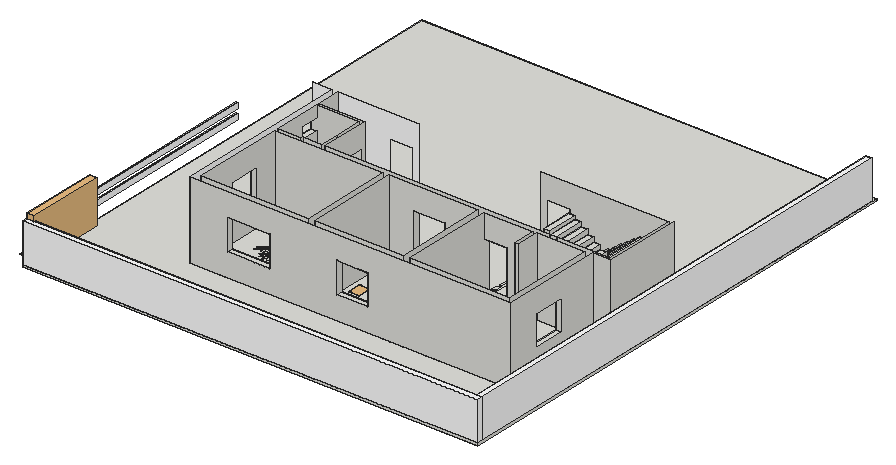
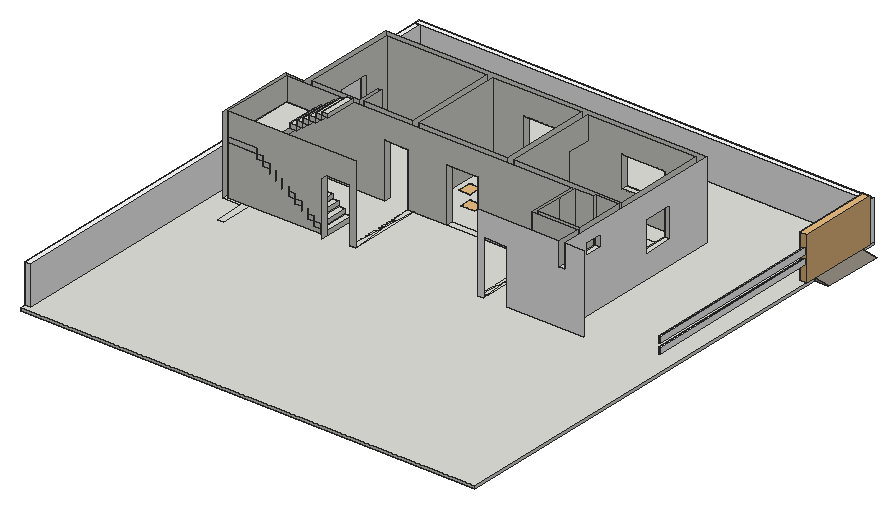
# SketchUp Ruby script. Lengths in inches.
U = 1.inch
M = Sketchup.active_model
def pt(a) = Geom::Point3d.new(a.map { |v| v * U })
def face(e, loops, mat)
  f = e.add_face(loops[0].map { |a| pt(a) })
  loops[1..].each { |l| e.add_face(l.map { |a| pt(a) }).erase! }
  f.material = f.back_material = mat if mat
  f
end
# faces: each face lists its corners as indices into pts; further lists are holes
def faces(e, pts, list, mat = nil) = list.each { |f| face(e, (f[0].is_a?(Array) ? f : [f]).map { |l| l.map { |i| pts[i] } }, mat) }
# xy, xz, yz: faces in a plane at the given z, y or x. An outline is a flat list of corners, or four numbers for a rectangle; further outlines are holes
def ring(l) = l.size == 4 ? [[l[0], l[1]], [l[2], l[1]], [l[2], l[3]], [l[0], l[3]]] : l.each_slice(2).to_a
def flat(e, list, mat, &to3) = list.each { |f| face(e, (f[0].is_a?(Array) ? f : [f]).map { |l| ring(l).map { |u, v| to3.(u, v) } }, mat) }
def xy(e, z, list, mat = nil) = flat(e, list, mat) { |x, y| [x, y, z] }
def xz(e, y, list, mat = nil) = flat(e, list, mat) { |x, z| [x, y, z] }
def yz(e, x, list, mat = nil) = flat(e, list, mat) { |y, z| [x, y, z] }
def lines(e, pts, list) = list.each { |a, b| e.add_line(pt(pts[a]), pt(pts[b])) }
# prism: a flat outline (further loops are holes) pulled along v
def prism(e, loops, v, mat = nil)
  f = face(e, loops, mat); d = Geom::Vector3d.new(v.map { |x| x * U })
  f.pushpull(f.normal.samedirection?(d) ? d.length : -d.length)
end
def box(e, o, s, mat = nil) = prism(e, [[o, [o[0] + s[0], o[1], o[2]], [o[0] + s[0], o[1] + s[1], o[2]], [o[0], o[1] + s[1], o[2]]]], [0, 0, s[2]], mat)
def at(x, y, z, deg = 0) = Geom::Transformation.translation(pt([x, y, z])) * Geom::Transformation.rotation(ORIGIN, Z_AXIS, deg.degrees)
def axes(o, x, y, z) = Geom::Transformation.new([*x, 0, *y, 0, *z, 0, *pt(o).to_a, 1])
def part(name) = M.definitions.add(name)
# library, detail: a bought-in or finely detailed component or shape, given as its bounding box
def library(name, o, s) = part(name).tap { |d| box(d.entities, o, s) }
def detail(e, o, s) = box(e.add_group.entities, o, s)
def put(e, d, t, mat = nil) = e.add_instance(d, t).tap { |i| i.material = mat if mat }
def group(e, t, mat = nil) = e.add_group.tap { |g| g.transformation = t; g.material = mat if mat }.entities
root = M.entities
M.materials.add("Manhattan Creative Coating MD 1125B 26.44cm").color = [255, 255, 255]
M.materials.add("Pp-1846-msg 17.72cm").color = [255, 255, 255]
M.materials.add("Tiles L02 200cm").color = [152, 144, 134]
c1 = library("Group\#36",[0,0,0],[178.08,17.07,78.35])
c2 = library("Chair - Desk\#3",[-10.5,-17,0],[21,17,0.01])
c3 = part("*U14\#2")
p = [[0,9.17,0],[-0.57,7.9375,0],[-1.06,6.67,0],[-1.46,5.37,0],[-1.77,4.05,0],[-1.99,2.71,0],
  [-2.13,1.36,0],[-2.17,0,0],[-2.13,-1.36,0],[-1.99,-2.71,0],[-1.77,-4.05,0],[-1.46,-5.37,0],
  [-1.06,-6.67,0],[-0.57,-7.9375,0],[0,-9.17,0],[0.57,-7.9375,0],[1.06,-6.67,0],[1.46,-5.37,0],
  [1.77,-4.05,0],[1.99,-2.71,0],[2.13,-1.36,0],[2.17,0,0],[2.13,1.36,0],[1.99,2.71,0],
  [1.77,4.05,0],[1.46,5.37,0],[1.06,6.67,0],[0.57,7.9375,0]]
lines(c3.entities,p,[[0,1],[1,2],[2,3],[3,4],[4,5],[5,6],[6,7],[7,8],[8,9],[9,10],[10,11],[11,12],
  [12,13],[13,14],[14,15],[15,16],[16,17],[17,18],[18,19],[19,20],[20,21],[21,22],[22,23],[23,24],
  [24,25],[25,26],[26,27],[27,0]])
c4 = part("*U15\#1")
put(c4.entities,c3,at(3814.69,2754.15,0))
put(c4.entities,c3,at(3810.96,2753.36,0,24))
put(c4.entities,c3,at(3807.875,2751.12,0,48))
put(c4.entities,c3,at(3805.97,2747.8125,0,72))
put(c4.entities,c3,at(3805.57,2744.02,0,96))
put(c4.entities,c3,at(3806.75,2740.39,0,120))
put(c4.entities,c3,at(3809.3,2737.56,0,144))
put(c4.entities,c3,at(3812.79,2736.01,0,168))
put(c4.entities,c3,at(3816.6,2736.01,0,-168))
put(c4.entities,c3,at(3820.09,2737.56,0,-144))
put(c4.entities,c3,at(3822.64,2740.39,0,-120))
put(c4.entities,c3,at(3823.82,2744.02,0,-96))
put(c4.entities,c3,at(3823.42,2747.8125,0,-72))
put(c4.entities,c3,at(3821.51,2751.12,0,-48))
put(c4.entities,c3,at(3818.42,2753.36,0,-24))
c5 = part("Group\#35")
box(c5.entities,[-3,0,0],[3,280.875,9])
c6 = library("*U30\#2",[-10.5,-33,0],[21,33,0.01])
c7 = part("Stair tread")
box(c7.entities,[0,0,0],[9.89,48,7])
c8 = part("Group\#5")
box(c8.entities,[108.84,0,77],[43.96,112.5,7])
xy(c8.entities,124,[[49.47,0,59.37,48]])
xz(c8.entities,48,[[49.47,119,59.37,124]])
yz(c8.entities,49.47,[[0,119,48,124]])
put(c8.entities,c7,at(9.89,64.5,7))
put(c8.entities,c7,at(19.79,64.5,14))
put(c8.entities,c7,at(0,64.5,0))
put(c8.entities,c7,at(29.68,64.5,21))
put(c8.entities,c7,at(39.58,64.5,28))
put(c8.entities,c7,at(49.47,64.5,35))
put(c8.entities,c7,at(89.05,64.5,63))
put(c8.entities,c7,at(89.05,0,91))
put(c8.entities,c7,at(79.16,0,98))
put(c8.entities,c7,at(98.95,64.5,70))
put(c8.entities,c7,at(69.26,0,105))
put(c8.entities,c7,at(79.16,64.5,56))
put(c8.entities,c7,at(59.37,64.5,42))
put(c8.entities,c7,at(69.26,64.5,49))
put(c8.entities,c7,at(98.95,0,84))
put(c8.entities,c7,at(59.37,0,112))
xy(root,0,[[178.31,129,178.31,199.58,187.31,199.58,187.31,138,236.56,138,236.56,129],[236.56,129,302.56,138],[302.56,129,302.56,138,502.31,138,502.31,282,481.31,282,481.31,291,511.31,291,511.31,138,667.31,138,667.31,175.67,676.31,175.67,676.31,129],[273.14,138,273.21,138,273.27,138.01,273.34,138.02,273.4,138.03,273.46,138.05,273.52,138.08,273.58,138.1,273.64,138.13,273.7,138.17,273.85,138.29,273.97,138.44,274.01,138.5,274.04,138.56,274.0625,138.62,274.09,138.68,274.11,138.74,274.12,138.8,274.13,138.87,274.14,138.93,274.14,167.08,274.13,167.17,274.09,167.35,274.07,167.4375,274.04,167.52,273.96,167.68,273.86,167.84,273.8,167.91,273.74,167.97,273.68,168.04,273.61,168.1,273.53,168.15,273.46,168.2,273.38,168.25,273.3,168.28,273.21,168.32,273.13,168.35,272.95,168.39,272.86,168.4,272.59,168.4,272.5,168.39,272.32,168.35,272.24,168.32,272.15,168.28,272.07,168.25,271.91,168.15,271.84,168.1,271.77,168.04,271.71,167.97,271.65,167.91,271.59,167.84,271.49,167.68,271.41,167.52,271.38,167.4375,271.35,167.35,271.33,167.26,271.32,167.17,271.3125,167.08,271.31,166.99,216.79,166.99,216.79,204.56,216.98,204.5625,217.17,204.58,217.36,204.61,217.55,204.65,217.73,204.71,218.09,204.85,218.26,204.94,218.42,205.04,218.58,205.15,218.73,205.27,218.875,205.4,219.01,205.54,219.13,205.6875,219.25,205.84,219.35,206,219.45,206.17,219.53,206.34,219.6,206.52,219.66,206.7,219.71,206.89,219.75,207.08,219.77,207.27,219.78,207.46,219.78,207.65,219.77,207.84,219.75,208.04,219.71,208.22,219.66,208.41,219.6,208.59,219.53,208.77,219.45,208.94,219.35,209.11,219.25,209.27,219.13,209.43,219.01,209.57,218.875,209.71,218.73,209.84,218.58,209.96,218.42,210.07,218.26,210.17,218.09,210.26,217.91,210.34,217.55,210.46,217.36,210.5,217.17,210.53,216.98,210.55,216.79,210.56,216.79,248.125,271.31,248.125,271.3125,248.03,271.32,247.94,271.33,247.85,271.35,247.76,271.38,247.68,271.41,247.59,271.49,247.43,271.54,247.35,271.59,247.28,271.71,247.14,271.77,247.08,271.91,246.96,271.99,246.91,272.15,246.83,272.24,246.79,272.32,246.77,272.41,246.74,272.5,246.73,272.59,246.71,272.86,246.71,272.95,246.73,273.04,246.74,273.13,246.77,273.21,246.79,273.3,246.83,273.46,246.91,273.53,246.96,273.61,247.02,273.68,247.08,273.74,247.14,273.86,247.28,273.91,247.35,273.96,247.43,274.04,247.59,274.07,247.68,274.09,247.76,274.13,247.94,274.14,248.03,274.14,281.07,274.13,281.13,274.12,281.2,274.11,281.26,274.09,281.32,274.0625,281.38,274.04,281.44,274.01,281.5,273.97,281.56,273.85,281.71,273.7,281.83,273.64,281.87,273.58,281.9,273.52,281.92,273.46,281.95,273.4,281.97,273.34,281.98,273.27,281.99,273.21,282,273.14,282,355.31,282,355.31,174,364.31,174,364.31,138],[645.22,168.15,654.6,182.11,654.6,176.02,665.48,176.02,665.48,195.21,655.11,195.21,655.11,199.87,665.48,199.87,665.48,219.06,655.11,219.06,655.11,226.15,667.17,226.15,667.17,168.15],
  [355.31,174,355.31,291,334.31,286.5,313.31,291,400.31,291,400.31,287,403.31,287,403.31,286,400.31,286,400.31,282,364.31,282,364.31,174],[667.31,175.67,676.31,226.67],[654.6,182.11,654.6,182.86,655.11,182.86],[640.18,182.86,640.02,183.42,639.96,183.66,640.32,183.29,640.74,182.86],[654.6,182.86,655.11,195.21],
  [639.96,183.66,639.8,183.82,639.73,183.99,639.51,184.55,639.29,185.12,639.06,185.6875,638.83,186.25,638.6,186.82,638.37,187.38,637.89,188.5,637.14,190.15,636.88,190.68,636.61,191.22,636.34,191.74,636.0625,192.26,635.78,192.77,635.18,193.77,634.875,194.25,634.56,194.72,634.23,195.18,633.89,195.63,633.55,196.07,633.19,196.49,632.83,196.9,632.45,197.3,632.0625,197.68,631.66,198.05,631.25,198.4,630.83,198.74,630.39,199.06,629.9375,199.36,629.47,199.64,628.99,199.9,628.5,200.15,627.99,200.37,627.47,200.57,626.93,200.76,626.38,200.93,625.82,201.08,625.25,201.22,624.68,201.35,623.52,201.59,622.94,201.7,622.36,201.8,621.22,202.02,620.65,202.14,620.1,202.26,619.55,202.39,619.02,202.53,618.51,202.6875,618.01,202.86,617.53,203.04,617.07,203.25,616.63,203.47,616.22,203.72,615.83,203.99,615.46,204.29,615.11,204.6,614.79,204.94,614.49,205.29,614.21,205.67,613.94,206.0625,613.7,206.47,613.48,206.91,613.27,207.36,613.08,207.82,612.91,208.3,612.76,208.8,612.62,209.3125,612.5,209.84,612.39,210.38,612.3,210.94,612.22,211.51,612.15,212.09,612.09,212.68,612.05,213.29,612.02,213.9,611.99,214.53,611.98,215.16,611.98,215.8,611.99,216.46,612,217.11,612.02,217.78,612.05,218.46,612.13,219.82,612.17,220.51,612.23,221.21,612.28,221.91,612.34,222.61,612.4,223.32,612.47,224.02,612.53,224.73,612.67,226.15,616.25,226.15,616.22,225.53,616.1,223.64,616.01,221.78,615.99,221.16,615.97,220.55,615.95,219.9375,615.94,219.33,615.94,218.14,615.95,217.55,615.99,216.39,616.03,215.82,616.07,215.26,616.125,214.7,616.1875,214.15,616.26,213.62,616.34,213.09,616.4375,212.57,616.55,212.06,616.67,211.56,616.8,211.07,616.95,210.59,617.11,210.125,617.29,209.67,617.49,209.23,617.69,208.8,617.92,208.39,618.16,207.98,618.42,207.6,618.7,207.22,619,206.87,619.32,206.52,619.65,206.2,620.01,205.89,620.39,205.6,620.78,205.32,621.2,205.06,621.63,204.81,622.08,204.57,623.02,204.13,623.51,203.92,624,203.72,625,203.32,626.02,202.93,627.55,202.33,628.05,202.12,628.54,201.9,629.03,201.67,629.5,201.43,629.96,201.18,630.41,200.92,630.85,200.64,631.27,200.35,631.67,200.04,632.07,199.72,632.45,199.38,632.8125,199.04,633.17,198.68,633.51,198.31,633.84,197.92,634.16,197.53,634.47,197.12,634.76,196.71,635.05,196.28,635.33,195.84,635.6,195.4,635.86,194.94,636.11,194.48,636.35,194.01,636.58,193.53,636.81,193.04,637.03,192.55,637.24,192.05,637.45,191.54,637.65,191.03,637.84,190.51,638.03,189.98,638.39,188.92,638.57,188.38,638.91,187.3,639.07,186.75,639.24,186.2,639.4,185.64,639.56,185.09,639.71,184.53,639.87,183.98],[178.31,199.58,187.31,247.58],[654.6,199.87,655.11,219.06],[667.31,226.67,667.31,291,700.11,291,700.11,403.5,667.31,403.5,667.31,453.9,676.31,453.9,676.31,408.16,704.78,408.16,704.78,287.13,676.31,287.13,676.31,226.67],[178.31,247.58,178.31,333.5,187.31,333.5,187.31,287,223.31,287,223.31,291,253.31,291,253.31,330.63,258.31,330.63,258.31,291,313.31,291,313.31,282,187.31,282,187.31,247.58],
  [666.73,259.11,666.58,259.16,666.52,259.2,666.5,259.22,666.47,259.24,666.43,259.28,666.41,259.31,666.39,259.33,666.37,259.36,666.36,259.39,666.34,259.42,666.32,259.48,666.32,259.51,666.3125,259.54,666.31,259.58,666.31,269.45,667.31,269.45,667.31,259.58,667.3,259.54,667.3,259.51,667.26,259.39,667.24,259.36,667.23,259.33,667.21,259.31,667.1875,259.28,667.17,259.26,667.14,259.24,667.12,259.22,667.09,259.2,667.07,259.18,667.04,259.16,666.89,259.11],[666.31,269.45,666.31,277.78,666.3125,277.81,666.32,277.84,666.32,277.87,666.34,277.93,666.36,277.96,666.37,277.99,666.39,278.02,666.41,278.04,666.43,278.07,666.45,278.09,666.47,278.12,666.5,278.14,666.52,278.16,666.55,278.17,666.58,278.1875,666.61,278.2,666.64,278.22,666.67,278.23,666.7,278.23,666.73,278.24,666.76,278.24,666.79,278.25,666.82,278.25,666.86,278.24,666.89,278.24,666.92,278.23,666.95,278.23,666.98,278.22,667.01,278.2,667.04,278.1875,667.07,278.17,667.09,278.16,667.12,278.14,667.17,278.09,667.1875,278.07,667.21,278.04,667.23,278.02,667.24,277.99,667.26,277.96,667.3,277.84,667.3,277.81,667.31,277.78,667.31,269.45],[313.31,282,313.31,291,334.31,286.5],[313.31,282,334.31,286.5,355.31,282],[355.31,282,334.31,286.5,355.31,291],
  [400.31,282,403.31,286],[403.31,282,451.31,291],[451.31,282,451.31,291,454.31,291,454.31,287,478.31,287,478.31,291,481.31,291,481.31,282,478.31,282,478.31,286,454.31,286,454.31,282],[454.31,282,478.31,286],[400.31,287,403.31,291],
  [454.31,287,478.31,291],[304.31,291,304.31,403.5,304.43,401.96,304.43,292.54],[304.31,291,304.43,292.54,304.43,291],[304.43,291,304.43,292.54,308.81,347.25,313.31,291],[313.31,291,308.81,347.25,313.31,403.5],
  [502.31,291,502.31,291.22,502.33,291.22],[502.31,291,502.33,291.22,511.29,291.22,511.31,291],[511.31,291,511.29,291.22,511.31,291.22],[502.31,291.22,502.31,403.5,506.81,347.25,502.33,291.22],[502.33,291.22,506.81,347.25,511.29,291.22],
  [511.29,291.22,506.81,347.25,511.31,403.5,511.31,291.22],[304.43,292.54,304.43,401.96,308.81,347.25],[178.31,333.5,178.31,367.5,258.31,367.5,258.31,362.5,187.31,362.5,187.31,333.5],[308.81,347.25,304.43,401.96,304.43,403.5,313.31,403.5],[506.81,347.25,502.31,403.5,511.31,403.5],
  [304.43,401.96,304.31,403.5,304.31,403.63,304.43,403.63],[304.43,403.5,313.31,403.63]])
xy(root,36,[[236.56,129,302.56,138],[406.31,129,454.31,138],[667.31,175.67,676.31,226.67],[178.31,199.58,187.31,247.58]])
xy(root,84,[[236.56,129,302.56,138],[406.31,129,454.31,138],[355.31,138,364.31,174],[667.31,175.67,676.31,226.67],[178.31,199.58,187.31,247.58],
  [403.31,282,451.31,291],[511.31,282,547.31,291],[253.31,330.63,258.31,362.5],[178.31,333.5,187.31,362.5],[178.31,367.5,187.31,403.63]])
xz(root,129,[[[178.31,0,676.31,120],[236.56,36,302.56,84],[406.31,36,454.31,84]]])
xz(root,138,[[[187.31,0,187.31,120,355.31,120,355.31,84,364.31,84,364.31,120,502.31,120,502.31,0],[236.56,36,302.56,84],[406.31,36,454.31,84]],[511.31,0,667.31,120]])
xz(root,174,[[355.31,0,364.31,84]])
xz(root,175.67,[[667.31,36,676.31,84]])
xz(root,199.58,[[178.31,36,187.31,84]])
xz(root,226.67,[[667.31,36,676.31,84]])
xz(root,247.1,[[587.97,0,592.97,120]])
xz(root,247.58,[[178.31,36,187.31,84]])
xz(root,282,[[187.31,0,355.31,120],[364.31,0,403.31,0,403.31,84,451.31,84,451.31,0,502.31,0,502.31,120,364.31,120],[547.31,0,587.97,0,587.97,120,511.31,120,511.31,84,547.31,84],[592.97,0,667.31,120]])
xz(root,287,[[187.31,0,223.31,120]])
xz(root,287.13,[[676.31,0,704.78,120]])
xz(root,291,[[223.31,0,253.31,120],[258.31,0,403.31,0,403.31,84,451.31,84,451.31,0,511.31,0,511.31,84,547.31,84,547.31,0,700.11,0,700.11,77,656.15,77,656.15,84,700.11,84,700.11,120,258.31,120],[656.15,77,700.11,84],[656.15,77,700.11,84]])
xz(root,330.63,[[253.31,0,258.31,84]])
xz(root,333.5,[[178.31,84,187.31,102]])
xz(root,362.5,[[187.31,0,258.31,0,258.31,84,253.31,84,253.31,120,187.31,120,187.31,102,178.31,102,178.31,84,187.31,84]])
xz(root,367.5,[[178.31,0,178.31,84,187.31,84,187.31,120,258.31,120,258.31,0]])
xz(root,403.5,[[502.31,0,511.31,0,511.31,84,547.31,84,547.31,0,700.11,0,700.11,120,502.31,120]])
xz(root,403.63,[[148.31,0,268.31,0,268.31,84,304.31,84,304.31,0,313.31,0,313.31,120,187.31,120,187.31,84,178.31,84,178.31,120,148.31,120]],"Pp-1846-msg 17.72cm")
yz(root,178.31,[[[129,0,129,120,403.63,120,403.63,84,367.5,84,367.5,0],[199.58,36,247.58,84],[333.5,84,362.5,102]]],"Pp-1846-msg 17.72cm")
yz(root,187.31,[[[138,0,282,120],[199.58,36,247.58,84]],[287,0,362.5,0,362.5,84,333.5,84,333.5,102,362.5,102,362.5,120,287,120],[367.5,84,403.63,120]])
yz(root,223.31,[[287,0,291,120]])
yz(root,236.56,[[129,36,138,84]])
yz(root,253.31,[[291,0,319.5,120],[319.5,0,319.5,120,362.5,120,362.5,84,330.63,84,330.63,0]])
yz(root,258.31,[[291,0,330.63,0,330.63,84,362.5,84,362.5,0,367.5,0,367.5,120,291,120]])
yz(root,302.56,[[129,36,138,84]])
yz(root,355.31,[[174,0,174,84,138,84,138,120,282,120,282,0]])
yz(root,364.31,[[174,0,282,0,282,120,138,120,138,84,174,84]])
yz(root,403.31,[[282,0,291,84]])
yz(root,406.31,[[129,36,138,84]])
yz(root,451.31,[[282,0,291,84]])
yz(root,454.31,[[129,36,138,84]])
yz(root,502.31,[[138,0,282,120]])
yz(root,511.31,[[138,0,291,0,291,84,282,84,282,120,138,120]])
yz(root,547.31,[[282,0,291,84],[403.5,0,412.5,84]])
yz(root,587.97,[[247.1,0,282,120]])
yz(root,592.97,[[247.1,0,282,120]])
yz(root,667.31,[[[138,0,282,120],[175.67,36,226.67,84]]])
yz(root,676.31,[[[129,0,287.13,120],[175.67,36,226.67,84]]])
yz(root,700.11,[[291,0,403.5,84],[291,77,403.5,84],[291,84,403.5,120]])
yz(root,704.78,[[287.13,0,408.16,120]])
g1 = group(root,at(22.31,0,0),"Pp-1846-msg 17.72cm")
box(g1,[0,0,0],[705,9,60])
g2 = group(root,at(0,6.92,-4),"Tiles L02 200cm")
prism(g2,[[[5.79,16.125,0],[22.31,16.125,0],[22.31,16.125,4],[0,16.125,0]]],[0,91.6,0])
put(root,c1,axes([21.73,130.21,-0.24],[0,-0.68389,0],[0.66,0,0],[0,0,0.86116]))
put(root,c2,axes([457.61,166.33,0],[1,0,0],[0,-1,0],[0,0,1]))
put(root,c2,at(493.2,204.24,0,-90))
put(root,c2,axes([372.1,204.24,0],[0,-1,0],[-1,0,0],[0,0,1]))
put(root,c4,at(-3571.25,-2537.01,0))
put(root,c2,at(457.61,242.43,0))
put(root,c2,axes([372.1,244.03,0],[0,-1,0],[-1,0,0],[0,0,1]))
put(root,c5,at(28.31,129,22.59),"Manhattan Creative Coating MD 1125B 26.44cm")
put(root,c5,at(28.31,129,37.59),"Manhattan Creative Coating MD 1125B 26.44cm")
put(root,c6,at(252.6,311.22,0,-90))
g3 = group(root,at(547.31,291,0))
xz(g3,0,[[49.47,119,59.37,124]])
g4 = group(g3,at(0,0,0))
put(g4,c7,at(9.89,64.5,7))
g5 = group(g4,at(0,0,0))
yz(g5,59.37,[[0,119,48,124]])
put(g5,c8,at(0,0,0))
g6 = group(root,at(148.31,129,-4))
box(g6,[-126,-129,0],[705,772.5,4])
g7 = group(root,at(718.31,78,0),"Pp-1846-msg 17.72cm")
box(g7,[0,-69,0],[9,754.5,60])
